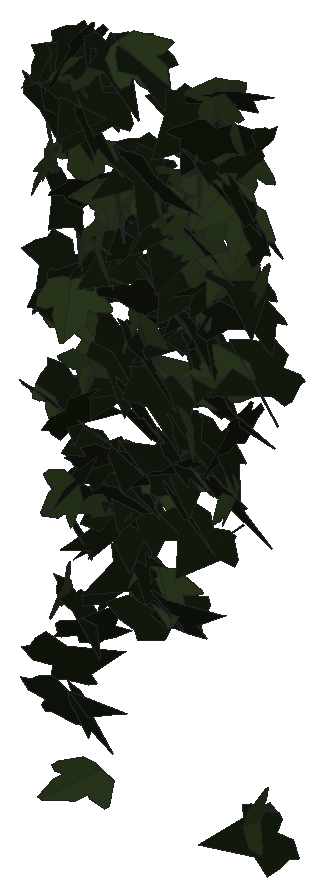
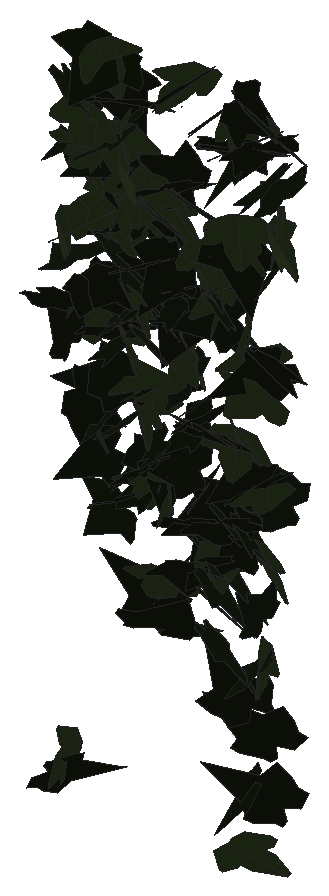
# SketchUp Ruby script. Lengths in inches.
U = 1.inch
M = Sketchup.active_model
def pt(a) = Geom::Point3d.new(a.map { |v| v * U })
def face(e, loops, mat)
  f = e.add_face(loops[0].map { |a| pt(a) })
  loops[1..].each { |l| e.add_face(l.map { |a| pt(a) }).erase! }
  f.material = f.back_material = mat if mat
  f
end
# faces: each face lists its corners as indices into pts; further lists are holes
def faces(e, pts, list, mat = nil) = list.each { |f| face(e, (f[0].is_a?(Array) ? f : [f]).map { |l| l.map { |i| pts[i] } }, mat) }
# xy, xz, yz: faces in a plane at the given z, y or x. An outline is a flat list of corners, or four numbers for a rectangle; further outlines are holes
def ring(l) = l.size == 4 ? [[l[0], l[1]], [l[2], l[1]], [l[2], l[3]], [l[0], l[3]]] : l.each_slice(2).to_a
def flat(e, list, mat, &to3) = list.each { |f| face(e, (f[0].is_a?(Array) ? f : [f]).map { |l| ring(l).map { |u, v| to3.(u, v) } }, mat) }
def xy(e, z, list, mat = nil) = flat(e, list, mat) { |x, y| [x, y, z] }
def xz(e, y, list, mat = nil) = flat(e, list, mat) { |x, z| [x, y, z] }
def yz(e, x, list, mat = nil) = flat(e, list, mat) { |y, z| [x, y, z] }
def lines(e, pts, list) = list.each { |a, b| e.add_line(pt(pts[a]), pt(pts[b])) }
# prism: a flat outline (further loops are holes) pulled along v
def prism(e, loops, v, mat = nil)
  f = face(e, loops, mat); d = Geom::Vector3d.new(v.map { |x| x * U })
  f.pushpull(f.normal.samedirection?(d) ? d.length : -d.length)
end
def box(e, o, s, mat = nil) = prism(e, [[o, [o[0] + s[0], o[1], o[2]], [o[0] + s[0], o[1] + s[1], o[2]], [o[0], o[1] + s[1], o[2]]]], [0, 0, s[2]], mat)
def at(x, y, z, deg = 0) = Geom::Transformation.translation(pt([x, y, z])) * Geom::Transformation.rotation(ORIGIN, Z_AXIS, deg.degrees)
def axes(o, x, y, z) = Geom::Transformation.new([*x, 0, *y, 0, *z, 0, *pt(o).to_a, 1])
def part(name) = M.definitions.add(name)
# library, detail: a bought-in or finely detailed component or shape, given as its bounding box
def library(name, o, s) = part(name).tap { |d| box(d.entities, o, s) }
def detail(e, o, s) = box(e.add_group.entities, o, s)
def put(e, d, t, mat = nil) = e.add_instance(d, t).tap { |i| i.material = mat if mat }
def group(e, t, mat = nil) = e.add_group.tap { |g| g.transformation = t; g.material = mat if mat }.entities
root = M.entities
M.materials.add("1026 AP 7946 SUNNY SIDE UP").color = [254, 231, 186]
M.materials.add("efeu1").color = [18, 25, 13]
M.materials.add("efeu2").color = [43, 57, 29]
c1 = part("ivyleaf_10")
p = [[0,0.5,-0.03],[-0.0625,2.02,-0.43],[-0.19,2.01,-0.46],[-0.54,1.05,-0.29],[-0.52,0.625,-0.18],[-0.83,0.76,-0.28],
  [-1.16,0.64,-0.33],[-1.15,0.33,-0.24],[-0.77,-0.39,0.02],[-0.3,-0.51,0.16],[0.04,-0.48,0.23],[-0.02,2.01,-0.4375],
  [-0.06,2.01,-0.43],[0.04,-0.49,0.23],[0.67,-0.49,0.14],[1.38,0.36,-0.2],[1.375,0.51,-0.24],[0.81,0.65,-0.19],
  [0.62,0.59,-0.15],[0.6,1.09,-0.28],[0.5,1.23,-0.31]]
faces(c1.entities,p,[[0,1,2,3,4,5,6,7,8,9,10],[11,12,0,13,14,15,16,17,18,19,20]],"efeu2")
c2 = part("ivyleaf_9")
p = [[1.54,2.16,1.25],[1.36,2.04,1.19],[-0.21,0.99,0.68],[-0.71,1.11,0.82],[-0.85,0.86,0.67],[-0.8,0.17,0.21],
  [-0.9,-0.01,0.1],[-0.67,-0.16,-0.02],[-0.08,-0.08,-0.05],[-0.03,-0.6,-0.4],[0.65,-0.88,-0.66],[0.83,-0.6,-0.49],
  [1.29,-0.42,-0.43],[1.8125,-0.07,-0.26],[1.21,0.44,0.15]]
faces(c2.entities,p,[[0,1,2,3,4,5,6,7,8,9,10,11,12,13,14]],"efeu1")
put(root,c1,axes([124.42,212.54,277.53],[0.12316,-0.29107,0.07806],[0.00734,-0.07882,-0.31058],[0.47353,0.07693,-0.01549]),"1026 AP 7946 SUNNY SIDE UP")
put(root,c1,axes([124.35,212.81,273.875],[0.25292,0.22521,-0.06282],[-0.02939,-0.06294,-0.28467],[-0.36623,0.16058,-0.02054]),"1026 AP 7946 SUNNY SIDE UP")
put(root,c2,axes([124.53,212.82,275.87],[-0.44269,-0.04822,-0.09389],[0.14795,-0.0137,-0.29293],[0.06538,-0.29552,0.02712]),"1026 AP 7946 SUNNY SIDE UP")
put(root,c2,axes([124.23,212.67,278.23],[0.06483,-0.2635,0.15344],[0.07992,-0.14368,-0.27445],[0.47037,0.06073,0.02549]),"1026 AP 7946 SUNNY SIDE UP")
put(root,c2,axes([124.12,212.66,273.7],[0.30329,-0.16016,0.14268],[0.21913,-0.04661,-0.25408],[0.2519,0.23338,0.04924]),"1026 AP 7946 SUNNY SIDE UP")
put(root,c1,axes([124.47,212.4,277.72],[0.15783,-0.25291,-0.1574],[0.05601,0.16913,-0.26582],[0.46006,0.06617,0.08636]),"1026 AP 7946 SUNNY SIDE UP")
put(root,c2,axes([124.48,212.91,273.95],[-0.05732,-0.2829,0.03635],[-0.00012,-0.03718,-0.29403],[0.44861,-0.03616,0.00457]),"1026 AP 7946 SUNNY SIDE UP")
put(root,c2,axes([124.53,212.78,276.76],[-0.06523,-0.16198,0.25578],[-0.07143,-0.24521,-0.17343],[0.46186,-0.0608,0.00931]),"1026 AP 7946 SUNNY SIDE UP")
put(root,c2,axes([124.4,212.74,278.38],[0.17277,-0.29324,0.00275],[-0.00666,-0.00622,-0.32258],[0.4611,0.10979,-0.00569]),"1026 AP 7946 SUNNY SIDE UP")
put(root,c2,axes([124.5,212.46,275.5625],[0.05717,0.03596,-0.31059],[-0.06643,0.30149,0.03354],[0.47309,0.03799,0.04224]),"1026 AP 7946 SUNNY SIDE UP")
put(root,c2,axes([124.28,212.65,269.18],[0.13987,-0.0573,0.27475],[0.39302,-0.09609,-0.10758],[0.17305,0.26454,0.02226]),"1026 AP 7946 SUNNY SIDE UP")
put(root,c2,axes([124.42,212.85,272],[0.11857,-0.19538,0.19268],[0.08533,-0.18046,-0.21653],[0.41787,0.09229,-0.01046]),"1026 AP 7946 SUNNY SIDE UP")
put(root,c2,axes([124.52,212.72,278.9375],[-0.03219,-0.28294,-0.13849],[0.01173,0.13263,-0.29146],[0.49133,-0.0217,-0.00212]),"1026 AP 7946 SUNNY SIDE UP")
put(root,c2,axes([124.9,212.55,279.28],[-0.4302,0.12308,-0.07879],[0.08376,-0.06813,-0.30684],[-0.21253,-0.27599,0.03857]),"1026 AP 7946 SUNNY SIDE UP")
put(root,c1,axes([124.76,212.36,271.17],[0.03226,-0.21172,-0.22694],[-0.0032,0.21949,-0.21742],[0.47905,0.01572,0.01383]),"1026 AP 7946 SUNNY SIDE UP")
put(root,c1,axes([124.84,212.36,272.64],[0.31417,-0.19601,-0.13394],[-0.1621,0.07873,-0.2875],[0.33136,0.22436,-0.01365]),"1026 AP 7946 SUNNY SIDE UP")
put(root,c1,axes([124.76,212.72,276.19],[-0.15115,0.28167,-0.03109],[-0.05385,-0.04485,-0.30308],[-0.44245,-0.09076,0.04751]),"1026 AP 7946 SUNNY SIDE UP")
put(root,c1,axes([124.48,212.77,275.21],[0.35989,0.05518,0.2118],[0.31513,0.04454,-0.24227],[-0.11142,0.30421,-0.00107]),"1026 AP 7946 SUNNY SIDE UP")
put(root,c1,axes([124.98,212.62,268.29],[0.24952,0.10593,-0.23794],[-0.30892,-0.12266,-0.19722],[-0.25474,0.25251,0.0061]),"1026 AP 7946 SUNNY SIDE UP")
put(root,c1,axes([124.85,212.79,277.64],[-0.36361,-0.20258,0.02079],[0.05048,-0.06812,-0.30825],[0.31629,-0.22201,0.0731]),"1026 AP 7946 SUNNY SIDE UP")
put(root,c2,axes([124.72,212.66,269.33],[0.31066,-0.15217,-0.15086],[-0.17982,0.09009,-0.25638],[0.27806,0.22828,0.00275]),"1026 AP 7946 SUNNY SIDE UP")
put(root,c1,axes([124.79,212.46,275.6],[0.29451,0.25694,-0.07331],[-0.04864,-0.06722,-0.32762],[-0.417,0.1893,-0.01356]),"1026 AP 7946 SUNNY SIDE UP")
put(root,c2,axes([124.97,212.62,277.25],[0.10549,0.28175,-0.08576],[-0.02561,-0.08334,-0.29884],[-0.46197,0.06896,-0.00302]),"1026 AP 7946 SUNNY SIDE UP")
put(root,c2,axes([124.5625,212.43,269.91],[-0.00585,-0.02548,0.28851],[0.43227,-0.05996,-0.00221],[0.09415,0.27374,0.02806]),"1026 AP 7946 SUNNY SIDE UP")
put(root,c2,axes([124.94,212.7,279.41],[-0.1538,0.09126,-0.29301],[0.22171,-0.25034,-0.13393],[-0.41493,-0.16759,0.03704]),"1026 AP 7946 SUNNY SIDE UP")
put(root,c2,axes([124.67,212.81,278.94],[0.07317,-0.30621,-0.0503],[0.0855,0.05495,-0.31244],[0.47958,0.03692,0.06338]),"1026 AP 7946 SUNNY SIDE UP")
put(root,c1,axes([124.95,212.72,274.42],[-0.45501,0.01314,0.00372],[-0.0075,-0.02751,-0.29721],[-0.02004,-0.28808,0.02685]),"1026 AP 7946 SUNNY SIDE UP")
put(root,c2,axes([124.87,212.32,273.88],[-0.05506,0.07566,-0.29925],[-0.11108,0.2826,0.08613],[0.4594,0.0774,-0.01504]),"1026 AP 7946 SUNNY SIDE UP")
put(root,c2,axes([124.76,212.63,270.92],[0.10457,-0.26318,0.09846],[0.04748,-0.09247,-0.28011],[0.43851,0.07277,0.00685]),"1026 AP 7946 SUNNY SIDE UP")
put(root,c1,axes([125,212.55,279.07],[-0.19615,-0.28348,-0.02949],[0.07576,0.00805,-0.31625],[0.4413,-0.12738,0.04119]),"1026 AP 7946 SUNNY SIDE UP")
put(root,c2,axes([125.08,212.5,273.12],[-0.28957,0.13493,-0.1719],[0.19111,-0.11685,-0.23513],[-0.27922,-0.2199,0.01734]),"1026 AP 7946 SUNNY SIDE UP")
put(root,c1,axes([124.91,212.74,274.58],[0.32135,-0.16768,0.12195],[0.12134,-0.09346,-0.272],[0.3,0.21742,-0.02061]),"1026 AP 7946 SUNNY SIDE UP")
put(root,c2,axes([125.1,212.6875,278.6875],[-0.39126,-0.19371,0.02762],[0.06576,-0.09674,-0.3081],[0.30063,-0.23095,0.10335]),"1026 AP 7946 SUNNY SIDE UP")
put(root,c2,axes([125.3,212.59,273.15],[-0.34172,0.17921,-0.0232],[0.00734,-0.03123,-0.28956],[-0.28411,-0.21635,0.02042]),"1026 AP 7946 SUNNY SIDE UP")
put(root,c2,axes([124.88,212.56,270.42],[0.34121,0.18674,0.04597],[-0.0741,-0.01184,0.29403],[0.29227,-0.22101,0.02087]),"1026 AP 7946 SUNNY SIDE UP")
put(root,c1,axes([125.11,212.75,277.16],[-0.37817,-0.17029,-0.06952],[0.10208,0.0232,-0.30288],[0.26874,-0.24845,0.01722]),"1026 AP 7946 SUNNY SIDE UP")
put(root,c2,axes([125.21,212.57,278.67],[-0.39545,-0.17904,-0.02082],[0.04609,-0.00816,-0.31716],[0.27937,-0.2521,0.02284]),"1026 AP 7946 SUNNY SIDE UP")
put(root,c2,axes([125.12,212.9,273.17],[-0.21209,-0.24598,-0.04981],[0.05689,0.03363,-0.28838],[0.38964,-0.1388,0.01499]),"1026 AP 7946 SUNNY SIDE UP")
put(root,c2,axes([125.38,212.71,276.42],[-0.36807,0.16862,-0.09481],[0.09321,-0.07615,-0.29645],[-0.28807,-0.24008,0.02521]),"1026 AP 7946 SUNNY SIDE UP")
put(root,c2,axes([125.44,212.66,271.33],[-0.29678,0.20939,-0.03644],[0.01721,-0.03926,-0.29005],[-0.33379,-0.1882,0.01745]),"1026 AP 7946 SUNNY SIDE UP")
put(root,c2,axes([125.11,212.34,278.46],[0.33093,-0.18795,-0.16548],[-0.20112,0.09611,-0.28988],[0.33142,0.246,-0.01068]),"1026 AP 7946 SUNNY SIDE UP")
put(root,c1,axes([125.16,212.65,276.66],[-0.10781,-0.20233,-0.23209],[0.20837,0.18637,-0.21398],[0.42662,-0.14215,0.04586]),"1026 AP 7946 SUNNY SIDE UP")
put(root,c2,axes([125.4375,212.67,272.21],[-0.26955,0.20508,-0.0971],[0.07715,-0.08316,-0.27543],[-0.3472,-0.1777,0.01418]),"1026 AP 7946 SUNNY SIDE UP")
put(root,c1,axes([125.33,212.47,276.38],[-0.17398,0.23969,0.19758],[-0.13385,0.17041,-0.27092],[-0.46237,-0.13952,0.00408]),"1026 AP 7946 SUNNY SIDE UP")
put(root,c1,axes([125.35,212.78,277.09],[-0.36459,-0.19249,0.04652],[0.01003,-0.07846,-0.3039],[0.31113,-0.22304,0.06431]),"1026 AP 7946 SUNNY SIDE UP")
put(root,c2,axes([125.34,212.93,274.48],[-0.3957,-0.12063,-0.06254],[0.12618,-0.03203,-0.28047],[0.17019,-0.25672,0.06252]),"1026 AP 7946 SUNNY SIDE UP")
put(root,c1,axes([125.35,212.5625,272.59],[-0.21744,-0.2469,-0.01605],[0.02162,0.00854,-0.29137],[0.38826,-0.13875,0.00724]),"1026 AP 7946 SUNNY SIDE UP")
put(root,c2,axes([125.53,212.89,274.5],[-0.45064,0.01345,0.0053],[-0.01244,-0.06306,-0.28865],[-0.01887,-0.27962,0.06363]),"1026 AP 7946 SUNNY SIDE UP")
put(root,c2,axes([125.12,212.82,279.27],[0.1303,-0.2986,-0.0299],[-0.00592,0.02732,-0.31906],[0.47145,0.08287,0.00426]),"1026 AP 7946 SUNNY SIDE UP")
put(root,c2,axes([124.99,212.72,276.1875],[0.39873,-0.12789,0.09642],[0.12753,-0.04857,-0.29278],[0.21487,0.26615,-0.00514]),"1026 AP 7946 SUNNY SIDE UP")
put(root,c2,axes([125.65,212.33,272.38],[-0.30013,0.26715,-0.01443],[-0.00968,-0.02345,-0.33784],[-0.42067,-0.19006,0.01807]),"1026 AP 7946 SUNNY SIDE UP")
put(root,c2,axes([125.13,212.46,273.21],[0.40107,0.09337,0.1205],[0.18602,0.0141,-0.27853],[-0.1431,0.28003,-0.02433]),"1026 AP 7946 SUNNY SIDE UP")
put(root,c2,axes([125.26,212.45,272.74],[0.45295,0.0809,-0.04448],[-0.05424,-0.03792,-0.30721],[-0.13397,0.28887,-0.02601]),"1026 AP 7946 SUNNY SIDE UP")
put(root,c1,axes([125.4,212.6875,277.2],[-0.18821,0.26457,-0.10896],[0.03056,-0.10849,-0.29865],[-0.44787,-0.11859,0.02541]),"1026 AP 7946 SUNNY SIDE UP")
put(root,c2,axes([125.3,212.89,275.01],[0.06345,-0.28999,0.00771],[-0.00789,-0.00992,-0.30161],[0.45613,0.04017,-0.00629]),"1026 AP 7946 SUNNY SIDE UP")
put(root,c2,axes([125.35,212.89,274.7],[-0.06559,-0.28661,0.03154],[0.00164,-0.03273,-0.2985],[0.4535,-0.04133,0.00564]),"1026 AP 7946 SUNNY SIDE UP")
put(root,c2,axes([125.81,212.47,276.72],[-0.09899,0.23715,0.2251],[-0.10643,0.20654,-0.25138],[-0.49428,-0.09197,0.00905]),"1026 AP 7946 SUNNY SIDE UP")
put(root,c2,axes([125.72,212.74,276.36],[-0.36601,-0.14744,0.11716],[-0.09791,-0.11131,-0.27857],[0.27679,-0.23434,0.05639]),"1026 AP 7946 SUNNY SIDE UP")
put(root,c2,axes([125.58,212.84,272.4],[-0.2049,-0.30484,-0.09136],[0.07187,0.07496,-0.34087],[0.49324,-0.13756,0.01172]),"1026 AP 7946 SUNNY SIDE UP")
put(root,c2,axes([125.68,212.84,272.99],[-0.31625,-0.20132,-0.03244],[0.07888,-0.00767,-0.2902],[0.31027,-0.20325,0.04072]),"1026 AP 7946 SUNNY SIDE UP")
put(root,c2,axes([125.9,212.85,277.81],[-0.47084,0.02592,-0.05816],[0.07171,-0.09795,-0.29533],[-0.06663,-0.28857,0.09313]),"1026 AP 7946 SUNNY SIDE UP")
put(root,c1,axes([125.78,212.68,275.51],[0.21062,-0.26717,0.0173],[-0.00324,-0.0215,-0.30779],[0.42107,0.13347,-0.01102]),"1026 AP 7946 SUNNY SIDE UP")
put(root,c2,axes([125.63,212.5,273.39],[0.25072,-0.21206,-0.13943],[-0.14041,0.10058,-0.27256],[0.36873,0.18249,-0.00898]),"1026 AP 7946 SUNNY SIDE UP")
put(root,c2,axes([126,212.46,271.87],[-0.418,0.09935,-0.01489],[0.00783,-0.0294,-0.29133],[-0.15781,-0.26463,0.02499]),"1026 AP 7946 SUNNY SIDE UP")
put(root,c1,axes([125.81,212.74,275.35],[-0.3726,0.17113,-0.02248],[0.00835,-0.03147,-0.30043],[-0.27134,-0.23597,0.02163]),"1026 AP 7946 SUNNY SIDE UP")
put(root,c2,axes([125.63,212.58,274.39],[0.34373,-0.18175,-0.07035],[-0.08737,0.03835,-0.29258],[0.29193,0.22548,-0.00473]),"1026 AP 7946 SUNNY SIDE UP")
put(root,c2,axes([125.53,212.83,273.8125],[0.31574,-0.15822,0.12684],[0.15244,-0.07735,-0.26382],[0.27693,0.22298,0.00061]),"1026 AP 7946 SUNNY SIDE UP")
put(root,c1,axes([125.72,212.55,279.48],[0.16151,0.27075,0.19142],[0.13077,0.16523,-0.29689],[-0.4981,0.13117,-0.01588]),"1026 AP 7946 SUNNY SIDE UP")
put(root,c1,axes([126.23,212.47,277.29],[-0.17286,0.07891,0.30952],[-0.45339,0.09138,-0.13308],[-0.17988,-0.30617,0.03798]),"1026 AP 7946 SUNNY SIDE UP")
put(root,c2,axes([125.72,212.8125,279.46],[0.09303,-0.30271,-0.06739],[-0.00406,0.06436,-0.31722],[0.48638,0.05843,0.01024]),"1026 AP 7946 SUNNY SIDE UP")
put(root,c2,axes([125.87,212.4375,276.05],[0.41698,0.1888,-0.06021],[-0.05181,-0.05601,-0.33461],[-0.30693,0.26595,-0.02532]),"1026 AP 7946 SUNNY SIDE UP")
put(root,c2,axes([125.68,212.77,275.04],[0.22155,-0.26686,0.09396],[0.04332,-0.09014,-0.31092],[0.44211,0.14256,-0.01662]),"1026 AP 7946 SUNNY SIDE UP")
put(root,c1,axes([126.01,212.84,273.26],[-0.09024,0.22627,-0.17139],[-0.01119,-0.17221,-0.23793],[-0.44267,-0.04177,0.04095]),"1026 AP 7946 SUNNY SIDE UP")
put(root,c2,axes([125.99,212.66,276.7],[0.4657,-0.04197,-0.11292],[-0.17615,-0.01447,-0.30687],[0.05389,0.31539,-0.02723]),"1026 AP 7946 SUNNY SIDE UP")
put(root,c2,axes([126.36,212.61,271.1],[-0.50347,-0.10613,0.07322],[0.09465,0.04563,0.3469],[-0.17774,0.32493,-0.02266]),"1026 AP 7946 SUNNY SIDE UP")
put(root,c2,axes([126.15,212.77,277.74],[-0.25652,-0.25706,0.04273],[-0.00104,-0.05024,-0.31279],[0.4098,-0.16104,0.02595]),"1026 AP 7946 SUNNY SIDE UP")
put(root,c2,axes([125.94,212.65,276.16],[0.36113,-0.19852,-0.0082],[-0.03367,-0.01437,-0.31177],[0.31052,0.22932,-0.02428]),"1026 AP 7946 SUNNY SIDE UP")
put(root,c2,axes([125.9,212.51,277.74],[0.21046,-0.12454,0.25473],[0.25656,-0.18737,-0.18877],[0.35293,0.21047,-0.01468]),"1026 AP 7946 SUNNY SIDE UP")
put(root,c2,axes([126.15,212.4,271.9],[0.21976,-0.21121,-0.1355],[-0.13256,0.10028,-0.25997],[0.36705,0.16267,-0.01276]),"1026 AP 7946 SUNNY SIDE UP")
put(root,c2,axes([126.43,212.52,273.375],[-0.12364,0.08827,0.27886],[-0.29855,-0.22492,0.01745],[0.33259,-0.16909,0.11934]),"1026 AP 7946 SUNNY SIDE UP")
put(root,c2,axes([126.48,212.83,275.52],[-0.40335,0.1147,-0.0762],[0.0803,-0.06683,-0.2871],[-0.19961,-0.25866,0.03847]),"1026 AP 7946 SUNNY SIDE UP")
put(root,c2,axes([126.45,212.36,273.51],[0.09532,0.28084,-0.01435],[0.00342,-0.01635,-0.29603],[-0.44226,0.0604,-0.00538]),"1026 AP 7946 SUNNY SIDE UP")
put(root,c1,axes([126.28,212.59,277.47],[0.39514,0.17563,0.02338],[0.02067,0.01906,-0.31563],[-0.2775,0.25151,0.00979]),"1026 AP 7946 SUNNY SIDE UP")
put(root,c2,axes([126.5,212.71,277.38],[-0.44567,0.0045,-0.12238],[0.17031,-0.11695,-0.27142],[-0.07714,-0.28421,0.1078]),"1026 AP 7946 SUNNY SIDE UP")
put(root,c2,axes([126.25,212.62,274.66],[-0.08517,-0.29134,-0.07098],[0.06211,0.06077,-0.30365],[0.46603,-0.06134,0.0275]),"1026 AP 7946 SUNNY SIDE UP")
put(root,c1,axes([126.46,212.77,277.72],[-0.47131,-0.07108,-0.00894],[0.02422,-0.0293,-0.3158],[0.10989,-0.29842,0.03127]),"1026 AP 7946 SUNNY SIDE UP")
put(root,c1,axes([126.3,212.46,271.78],[0.3917,0.11892,0.07195],[0.11156,0.01153,-0.28359],[-0.18533,0.25828,-0.01863]),"1026 AP 7946 SUNNY SIDE UP")
put(root,c2,axes([126.46,212.59,277.05],[-0.39272,-0.09657,-0.14142],[0.22203,0.01035,-0.27319],[0.14136,-0.28455,0.0362]),"1026 AP 7946 SUNNY SIDE UP")
put(root,c1,axes([126.375,212.61,273.3],[0.32728,0.19663,0.02326],[0.05346,-0.00487,-0.29371],[-0.30639,0.20919,-0.0264]),"1026 AP 7946 SUNNY SIDE UP")
put(root,c2,axes([126.8,212.55,277.37],[-0.07479,0.1789,0.25162],[-0.23534,0.19988,-0.18043],[-0.41233,-0.14653,0.05734]),"1026 AP 7946 SUNNY SIDE UP")
put(root,c1,axes([126.18,212.72,274.74],[0.21469,0.01282,0.2641],[0.36973,0.10999,-0.13407],[-0.16155,0.26875,0.04411]),"1026 AP 7946 SUNNY SIDE UP")
put(root,c2,axes([126.4,212.87,273.53],[-0.06414,-0.28507,0.0091],[0.00094,-0.01065,-0.29673],[0.44855,-0.04074,0.00193]),"1026 AP 7946 SUNNY SIDE UP")
put(root,c2,axes([126.38,212.53,273.77],[0.34317,-0.12104,-0.14749],[-0.15587,0.11076,-0.25272],[0.24923,0.23593,0.04503]),"1026 AP 7946 SUNNY SIDE UP")
put(root,c2,axes([126.77,212.4375,276.125],[-0.16836,0.27825,0.00592],[-0.05176,-0.00823,-0.30522],[-0.43449,-0.10683,0.03407]),"1026 AP 7946 SUNNY SIDE UP")
put(root,c2,axes([126.62,212.74,276.4],[-0.26497,-0.23008,0.11111],[-0.00244,-0.12996,-0.28543],[0.40042,-0.15304,0.07179]),"1026 AP 7946 SUNNY SIDE UP")
put(root,c1,axes([126.65,212.87,277.89],[0.14122,-0.24887,0.15658],[0.05754,-0.14965,-0.27305],[0.45608,0.09594,-0.01404]),"1026 AP 7946 SUNNY SIDE UP")
put(root,c1,axes([126.7,212.76,276.01],[0.37244,-0.1839,-0.03193],[-0.05126,0.00679,-0.30852],[0.28846,0.23865,-0.0136]),"1026 AP 7946 SUNNY SIDE UP")
put(root,c1,axes([126.67,212.77,277.32],[-0.05509,-0.22002,0.21624],[0.08241,-0.21372,-0.22171],[0.47236,0.01162,0.0639]),"1026 AP 7946 SUNNY SIDE UP")
put(root,c2,axes([126.34,212.4,271.35],[0.38128,0.07101,-0.14209],[0.19487,0.06651,0.25936],[0.14766,-0.27113,0.02462]),"1026 AP 7946 SUNNY SIDE UP")
put(root,c1,axes([126.7,212.47,274.25],[0.32222,-0.19036,-0.07676],[-0.00798,0.09928,-0.27916],[0.32072,0.19372,0.07017]),"1026 AP 7946 SUNNY SIDE UP")
put(root,c2,axes([126.8,212.78,278.84],[-0.40754,-0.16457,0.05439],[0.02081,-0.11528,-0.29868],[0.27141,-0.23827,0.10456]),"1026 AP 7946 SUNNY SIDE UP")
put(root,c2,axes([126.51,212.5,273.15],[0.3279,-0.21081,-0.02944],[-0.05348,0.00477,-0.3047],[0.32995,0.21027,-0.02013]),"1026 AP 7946 SUNNY SIDE UP")
put(root,c1,axes([126.7,212.82,275.36],[0.27874,-0.22399,0.08453],[0.08601,-0.06297,-0.29462],[0.36581,0.18548,0.00486]),"1026 AP 7946 SUNNY SIDE UP")
put(root,c2,axes([126.57,212.68,275.89],[0.14695,-0.26496,0.11431],[0.03004,-0.11227,-0.2895],[0.4516,0.09369,-0.01794]),"1026 AP 7946 SUNNY SIDE UP")
put(root,c2,axes([126.95,212.74,276.24],[-0.04413,0.19191,-0.23926],[0.01846,-0.23347,-0.20064],[-0.47469,-0.02692,0.01444]),"1026 AP 7946 SUNNY SIDE UP")
put(root,c1,axes([126.95,212.74,278.28],[-0.46087,-0.08907,0.04122],[-0.03622,-0.06155,-0.31141],[0.14954,-0.28941,0.05161]),"1026 AP 7946 SUNNY SIDE UP")
put(root,c2,axes([126.66,212.68,274.15],[0.17153,-0.27239,-0.05339],[0.00499,0.05526,-0.30102],[0.43551,0.10665,0.02447]),"1026 AP 7946 SUNNY SIDE UP")
put(root,c2,axes([127.16,212.51,276.43],[-0.29543,0.22851,0.02356],[-0.0599,-0.00356,-0.30304],[-0.35591,-0.18908,0.03145]),"1026 AP 7946 SUNNY SIDE UP")
put(root,c2,axes([126.72,212.83,275.7],[0.06268,-0.27071,0.09886],[0.01128,-0.09747,-0.28238],[0.4523,0.03995,-0.00666]),"1026 AP 7946 SUNNY SIDE UP")
put(root,c2,axes([126.74,212.77,275.3125],[0.21811,-0.26384,-0.01046],[-0.02519,0.00135,-0.30675],[0.41431,0.13898,-0.01314]),"1026 AP 7946 SUNNY SIDE UP")
put(root,c1,axes([127.08,212.51,277],[-0.37463,-0.17012,0.08973],[-0.07799,-0.08096,-0.29984],[0.29094,-0.24076,0.03516]),"1026 AP 7946 SUNNY SIDE UP")
put(root,c1,axes([126.83,212.68,278.23],[0.13164,-0.20624,0.22152],[0.22512,-0.16938,-0.22456],[0.41237,0.1583,0.05188]),"1026 AP 7946 SUNNY SIDE UP")
put(root,c2,axes([127,212.81,275.41],[-0.26785,-0.23407,0.00742],[0.03576,-0.02703,-0.29629],[0.36655,-0.1684,0.03433]),"1026 AP 7946 SUNNY SIDE UP")
put(root,c2,axes([126.8,212.64,278.41],[0.34527,-0.19497,-0.12447],[-0.07043,0.12608,-0.29545],[0.35279,0.21599,0.06283]),"1026 AP 7946 SUNNY SIDE UP")
put(root,c1,axes([127,212.45,277.36],[-0.41663,-0.12422,-0.0791],[0.12891,0.00336,-0.29979],[0.18933,-0.27565,0.03005]),"1026 AP 7946 SUNNY SIDE UP")
put(root,c2,axes([127.05,212.6,272.73],[-0.26086,-0.22448,0.11068],[-0.01338,-0.12539,-0.28086],[0.39196,-0.15368,0.06407]),"1026 AP 7946 SUNNY SIDE UP")
put(root,c2,axes([126.8125,212.4375,277.14],[0.43,-0.12621,-0.00847],[-0.0254,-0.01715,-0.30952],[0.19717,0.27303,-0.02141]),"1026 AP 7946 SUNNY SIDE UP")
put(root,c1,axes([127.19,212.73,279.37],[-0.17262,-0.27769,0.10746],[-0.01499,-0.10953,-0.30674],[0.46707,-0.10615,0.02987]),"1026 AP 7946 SUNNY SIDE UP")
put(root,c1,axes([127.19,212.64,277.84],[-0.44643,-0.10531,0.02834],[-0.01573,-0.05291,-0.30866],[0.17066,-0.28035,0.04568]),"1026 AP 7946 SUNNY SIDE UP")
put(root,c2,axes([127.13,212.43,272.53],[0.16361,0.16458,0.21993],[0.0825,0.2111,-0.19362],[-0.41457,0.10696,0.04827]),"1026 AP 7946 SUNNY SIDE UP")
put(root,c2,axes([127.28,212.4,278.92],[0.14326,0.20433,-0.22614],[-0.09863,-0.2126,-0.23072],[-0.4625,0.10863,-0.02085]),"1026 AP 7946 SUNNY SIDE UP")
put(root,c2,axes([127.27,212.83,276.0625],[-0.07825,0.13257,-0.26317],[0.07245,-0.253,-0.14556],[-0.44777,-0.0641,0.02244]),"1026 AP 7946 SUNNY SIDE UP")
put(root,c2,axes([126.89,212.62,277.98],[0.44677,-0.13548,0.02926],[0.02108,-0.03937,-0.32307],[0.21689,0.2829,-0.02888]),"1026 AP 7946 SUNNY SIDE UP")
put(root,c2,axes([126.83,212.72,274.63],[0.35594,-0.1246,0.13813],[0.18199,-0.06921,-0.26656],[0.22402,0.2542,-0.00292]),"1026 AP 7946 SUNNY SIDE UP")
put(root,c2,axes([127.15,212.55,279.34],[0.36388,0.20762,0.04633],[-0.00469,0.06798,-0.31536],[-0.33361,0.2255,0.05497]),"1026 AP 7946 SUNNY SIDE UP")
put(root,c2,axes([127.03,212.84,274.04],[0.10719,-0.27044,0.08392],[0.00431,-0.08474,-0.28726],[0.44479,0.06599,-0.01744]),"1026 AP 7946 SUNNY SIDE UP")
put(root,c1,axes([127.29,212.58,277.96],[0.4293,0.11034,-0.13725],[-0.18371,-0.06753,-0.30325],[-0.20162,0.29647,-0.01592]),"1026 AP 7946 SUNNY SIDE UP")
put(root,c1,axes([127.61,212.52,275.26],[-0.15524,0.00749,0.2834],[-0.38089,-0.14096,-0.08645],[0.2052,-0.25599,0.05394]),"1026 AP 7946 SUNNY SIDE UP")
put(root,c1,axes([127.15,212.59,279.23],[-0.32858,0.16367,-0.17149],[0.18906,-0.11749,-0.27367],[-0.31586,-0.24059,0.01458]),"1026 AP 7946 SUNNY SIDE UP")
put(root,c2,axes([127.38,212.97,274.4],[-0.18806,0.08907,-0.32582],[0.27687,-0.26742,-0.14751],[-0.43711,-0.2077,0.04675]),"1026 AP 7946 SUNNY SIDE UP")
put(root,c1,axes([127.42,212.78,278.41],[-0.47737,0.06109,-0.00294],[-0.01301,-0.05709,-0.31379],[-0.09531,-0.29819,0.0576]),"1026 AP 7946 SUNNY SIDE UP")
put(root,c2,axes([127.14,212.57,273.44],[0.43958,-0.10784,0.00278],[-0.01123,-0.02768,-0.30746],[0.16928,0.2782,-0.02763]),"1026 AP 7946 SUNNY SIDE UP")
put(root,c1,axes([127.52,212.58,276.89],[-0.18262,-0.22832,0.18382],[-0.03955,-0.18493,-0.25985],[0.45518,-0.10767,0.05117]),"1026 AP 7946 SUNNY SIDE UP")
put(root,c1,axes([127.55,212.38,273.5625],[0.2292,-0.27129,-0.08235],[-0.06892,0.06542,-0.3168],[0.43865,0.15203,-0.00674]),"1026 AP 7946 SUNNY SIDE UP")
put(root,c2,axes([127.9,212.41,277.74],[0.00905,0.00932,-0.34945],[-0.53365,0.00132,-0.00589],[0.00183,0.33931,0.01161]),"1026 AP 7946 SUNNY SIDE UP")
put(root,c2,axes([127.85,212.61,278.72],[-0.30618,0.24322,-0.02966],[0.00588,-0.03559,-0.32057],[-0.38533,-0.1938,0.01868]),"1026 AP 7946 SUNNY SIDE UP")
put(root,c2,axes([127.47,212.73,276.72],[-0.03923,-0.30094,0.04465],[0.04792,-0.04744,-0.3094],[0.47606,-0.02003,0.03483]),"1026 AP 7946 SUNNY SIDE UP")
put(root,c2,axes([127.49,212.86,276.28],[-0.01122,-0.27857,0.09132],[0.15221,-0.08742,-0.27069],[0.43454,0.02343,0.09718]),"1026 AP 7946 SUNNY SIDE UP")
put(root,c1,axes([127.67,212.54,277.73],[0.47433,-0.06838,0.02619],[0.02977,-0.03273,-0.31757],[0.11101,0.30099,-0.02672]),"1026 AP 7946 SUNNY SIDE UP")
put(root,c2,axes([127.59,212.42,278.1],[0.33515,-0.20752,-0.09427],[-0.09582,0.06688,-0.30603],[0.34274,0.22163,0.00663]),"1026 AP 7946 SUNNY SIDE UP")
put(root,c1,axes([127.74,212.86,276.6875],[0.13363,-0.25721,0.1251],[0.12529,-0.10169,-0.27662],[0.43036,0.10947,0.04169]),"1026 AP 7946 SUNNY SIDE UP")
put(root,c1,axes([127.91,212.43,268.64],[-0.01024,0.07184,0.35274],[-0.19698,0.31884,-0.06959],[-0.51297,-0.12387,0.01968]),"1026 AP 7946 SUNNY SIDE UP")
put(root,c2,axes([128,212.74,268.42],[-0.00118,-0.16244,-0.25955],[-0.02261,-0.25071,0.16571],[-0.46959,0.01248,-0.00733]),"1026 AP 7946 SUNNY SIDE UP")
put(root,c2,axes([127.62,212.83,275.01],[0.09377,-0.16255,0.24344],[0.09152,-0.23044,-0.17909],[0.44284,0.08205,-0.01454]),"1026 AP 7946 SUNNY SIDE UP")
put(root,c2,axes([128.09,212.74,275.47],[-0.4214,-0.07585,0.09137],[-0.12457,-0.04633,-0.28632],[0.13544,-0.2786,0.02094]),"1026 AP 7946 SUNNY SIDE UP")
